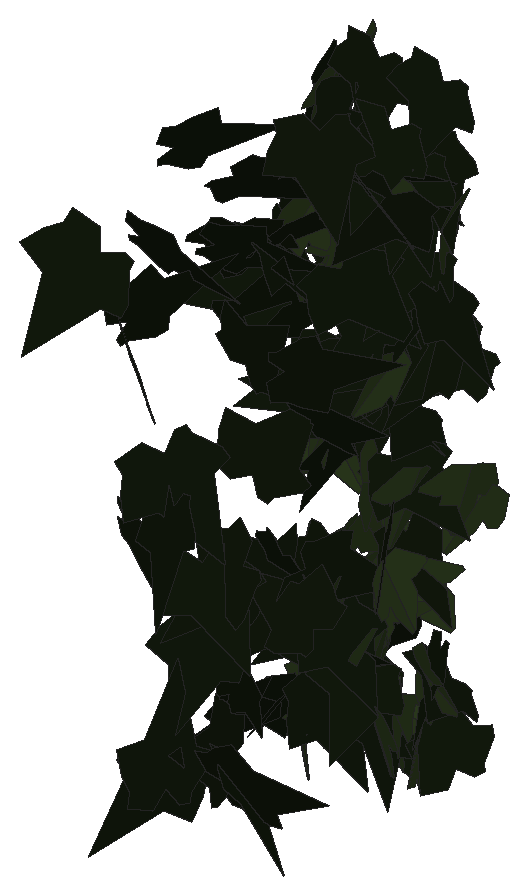
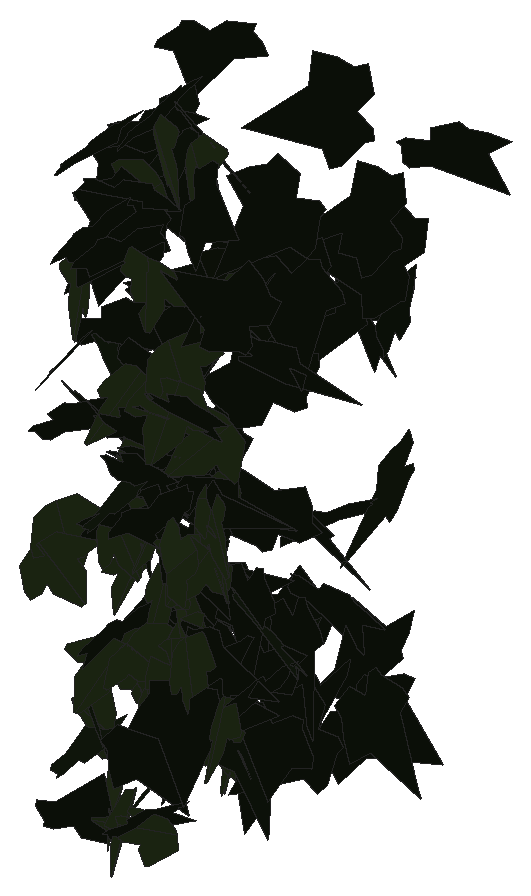
# SketchUp Ruby script. Lengths in inches.
U = 1.inch
M = Sketchup.active_model
def pt(a) = Geom::Point3d.new(a.map { |v| v * U })
def face(e, loops, mat)
  f = e.add_face(loops[0].map { |a| pt(a) })
  loops[1..].each { |l| e.add_face(l.map { |a| pt(a) }).erase! }
  f.material = f.back_material = mat if mat
  f
end
# faces: each face lists its corners as indices into pts; further lists are holes
def faces(e, pts, list, mat = nil) = list.each { |f| face(e, (f[0].is_a?(Array) ? f : [f]).map { |l| l.map { |i| pts[i] } }, mat) }
# xy, xz, yz: faces in a plane at the given z, y or x. An outline is a flat list of corners, or four numbers for a rectangle; further outlines are holes
def ring(l) = l.size == 4 ? [[l[0], l[1]], [l[2], l[1]], [l[2], l[3]], [l[0], l[3]]] : l.each_slice(2).to_a
def flat(e, list, mat, &to3) = list.each { |f| face(e, (f[0].is_a?(Array) ? f : [f]).map { |l| ring(l).map { |u, v| to3.(u, v) } }, mat) }
def xy(e, z, list, mat = nil) = flat(e, list, mat) { |x, y| [x, y, z] }
def xz(e, y, list, mat = nil) = flat(e, list, mat) { |x, z| [x, y, z] }
def yz(e, x, list, mat = nil) = flat(e, list, mat) { |y, z| [x, y, z] }
def lines(e, pts, list) = list.each { |a, b| e.add_line(pt(pts[a]), pt(pts[b])) }
# prism: a flat outline (further loops are holes) pulled along v
def prism(e, loops, v, mat = nil)
  f = face(e, loops, mat); d = Geom::Vector3d.new(v.map { |x| x * U })
  f.pushpull(f.normal.samedirection?(d) ? d.length : -d.length)
end
def box(e, o, s, mat = nil) = prism(e, [[o, [o[0] + s[0], o[1], o[2]], [o[0] + s[0], o[1] + s[1], o[2]], [o[0], o[1] + s[1], o[2]]]], [0, 0, s[2]], mat)
def at(x, y, z, deg = 0) = Geom::Transformation.translation(pt([x, y, z])) * Geom::Transformation.rotation(ORIGIN, Z_AXIS, deg.degrees)
def axes(o, x, y, z) = Geom::Transformation.new([*x, 0, *y, 0, *z, 0, *pt(o).to_a, 1])
def part(name) = M.definitions.add(name)
# library, detail: a bought-in or finely detailed component or shape, given as its bounding box
def library(name, o, s) = part(name).tap { |d| box(d.entities, o, s) }
def detail(e, o, s) = box(e.add_group.entities, o, s)
def put(e, d, t, mat = nil) = e.add_instance(d, t).tap { |i| i.material = mat if mat }
def group(e, t, mat = nil) = e.add_group.tap { |g| g.transformation = t; g.material = mat if mat }.entities
root = M.entities
M.materials.add("efeu1").color = [18, 25, 13]
M.materials.add("efeu2").color = [43, 57, 29]
c1 = part("ivyleaf_9")
p = [[1.54,2.16,1.25],[1.36,2.04,1.19],[-0.21,0.99,0.68],[-0.71,1.11,0.82],[-0.85,0.86,0.67],[-0.8,0.17,0.21],
  [-0.9,-0.01,0.1],[-0.67,-0.16,-0.02],[-0.08,-0.08,-0.05],[-0.03,-0.6,-0.4],[0.65,-0.88,-0.66],[0.83,-0.6,-0.49],
  [1.29,-0.42,-0.43],[1.8125,-0.07,-0.26],[1.21,0.44,0.15]]
faces(c1.entities,p,[[0,1,2,3,4,5,6,7,8,9,10,11,12,13,14]],"efeu1")
c2 = part("ivyleaf_10")
p = [[0,0.5,-0.03],[-0.0625,2.02,-0.43],[-0.19,2.01,-0.46],[-0.54,1.05,-0.29],[-0.52,0.625,-0.18],[-0.83,0.76,-0.28],
  [-1.16,0.64,-0.33],[-1.15,0.33,-0.24],[-0.77,-0.39,0.02],[-0.3,-0.51,0.16],[0.04,-0.48,0.23],[-0.02,2.01,-0.4375],
  [-0.06,2.01,-0.43],[0.04,-0.49,0.23],[0.67,-0.49,0.14],[1.38,0.36,-0.2],[1.375,0.51,-0.24],[0.81,0.65,-0.19],
  [0.62,0.59,-0.15],[0.6,1.09,-0.28],[0.5,1.23,-0.31]]
faces(c2.entities,p,[[0,1,2,3,4,5,6,7,8,9,10],[11,12,0,13,14,15,16,17,18,19,20]],"efeu2")
put(root,c1,axes([592.36,120.74,293.89],[-1.14457,0.06612,0.67883],[-0.67994,-0.00656,-1.1458],[-0.05352,-1.33072,0.03938]))
put(root,c1,axes([591.87,115.34,278.18],[-0.6134,1.00067,-0.76076],[0.3582,-0.67226,-1.17308],[-1.2049,-0.70929,0.03855]))
put(root,c2,axes([591.48,123.75,281.43],[0.25817,-0.97901,-0.59637],[0.14023,0.63368,-0.97957],[1.13774,0.14405,0.25606]))
put(root,c1,axes([591.9,111.61,298.5625],[-1.18923,-0.86005,0.10812],[-0.0968,-0.05064,-1.46755],[0.86139,-1.19306,-0.01565]))
put(root,c1,axes([592.14,119.23,296.43],[0.51316,1.03145,-0.63629],[-0.3835,-0.51727,-1.1478],[-1.14964,0.63295,0.09887]))
put(root,c1,axes([591.57,113.87,286.72],[1.18466,-0.50835,-0.63513],[-0.54554,0.33587,-1.28639],[0.60348,1.30154,0.0839]))
put(root,c1,axes([591.44,121.65,281.75],[0.54465,-0.90417,-0.67064],[-0.09148,0.707,-1.02748],[1.12201,0.49655,0.24178]))
put(root,c2,axes([592.77,122.97,288.59],[-0.65154,0.23488,0.97689],[-0.93643,0.27996,-0.69187],[-0.3641,-1.14036,0.03135]))
put(root,c1,axes([591.52,114.32,292.64],[-0.12498,-0.22861,1.35165],[0.38183,-1.30935,-0.18615],[1.3166,0.35803,0.18229]))
put(root,c1,axes([591.53,114.03,294.93],[0.43693,0.10982,1.41408],[1.05683,0.96162,-0.40122],[-0.94593,1.12509,0.2049]))
put(root,c1,axes([591.1,115.33,297.37],[1.16534,-0.32839,0.64756],[0.62053,-0.18536,-1.2107],[0.37699,1.32023,-0.00891]))
put(root,c1,axes([593.18,119.35,282.35],[-0.20471,0.90108,1.06087],[-0.70737,0.85614,-0.86368],[-1.19876,-0.65907,0.32848]))
put(root,c1,axes([592.625,114.95,277.32],[-0.06744,0.31516,-1.46174],[0.27376,-1.43589,-0.32222],[-1.47005,-0.28185,0.00705]))
put(root,c1,axes([593.2,123.18,289.14],[-1.02742,-0.18444,0.70049],[-0.69258,-0.10601,-1.04374],[0.21221,-1.23897,-0.01497]))
put(root,c2,axes([591.92,123.57,292.27],[-0.92808,-0.1007,-0.77885],[0.7694,0.12508,-0.93299],[0.15741,-1.20511,-0.03175]))
put(root,c1,axes([593.57,123.0625,288.75],[-0.81472,0.12778,0.98929],[-0.98397,0.10681,-0.82414],[-0.16381,-1.27713,0.03006]))
put(root,c1,axes([591.71,122.29,296.16],[0.21451,-0.10207,1.20924],[1.18259,-0.25797,-0.23156],[0.27231,1.20072,0.05304]))
put(root,c1,axes([592.15,120.32,292.25],[1.19976,0.61452,0.39653],[-0.38139,-0.12432,1.34661],[0.62403,-1.25746,0.06065]))
put(root,c1,axes([593.01,124.67,293.53],[-1.18188,-0.31478,-0.11874],[0.12949,-0.0253,-1.22173],[0.31051,-1.18756,0.0575]))
put(root,c1,axes([591.82,118.57,295.94],[1.10946,0.20211,0.77368],[0.74065,0.23905,-1.12455],[-0.30143,1.33129,0.08447]))
put(root,c1,axes([592.5,117.51,277.72],[0.60087,0.91157,0.89309],[0.51767,0.72816,-1.09151],[-1.16644,0.79274,-0.02436]))
put(root,c2,axes([592.72,125.05,287.43],[-0.29165,0.09054,-1.21967],[-0.07384,-1.25289,-0.07535],[-1.2208,0.05415,0.29594]))
put(root,c1,axes([593.89,122.01,282.14],[-0.5819,-0.01429,-1.14079],[-1.0494,-0.49574,0.5415],[-0.44762,1.18078,0.21353]))
put(root,c1,axes([593.09,123.7,281.29],[0.50094,1.04363,-0.38049],[-0.22491,-0.31346,-1.15588],[-1.08783,0.5454,0.06376]))
put(root,c1,axes([592.72,123.72,301.26],[-0.39489,0.23985,-1.23143],[0.90932,-0.83472,-0.45418],[-0.86435,-0.98773,0.08479]))
put(root,c2,axes([593.03,122.72,287.51],[0.92844,-0.7396,-0.28525],[-0.22808,0.17149,-1.18699],[0.75918,0.95601,-0.00776]))
put(root,c2,axes([592.6875,123.07,289.2],[-0.19418,-0.48725,1.13069],[0.48465,-1.0825,-0.38325],[1.13181,0.37994,0.3581]))
put(root,c1,axes([593,119.29,278.41],[0.68816,1.04968,-0.22079],[-0.12979,-0.17891,-1.25511],[-1.06477,0.70022,0.01029]))
put(root,c2,axes([593.11,121.79,296.25],[0.17074,0.86733,-0.87553],[-0.36793,-0.8077,-0.87189],[-1.17619,0.37857,0.14565]))
put(root,c1,axes([592.42,119.75,286.65],[-0.59776,0.14735,1.18784],[1.15522,-0.27647,0.61564],[0.31327,1.30071,-0.00371]))
put(root,c1,axes([592.6875,118.47,299.01],[0.91336,0.85435,0.43133],[0.28933,0.32184,-1.25016],[-0.91227,0.95744,0.03535]))
put(root,c1,axes([592.35,115.6,301.36],[0.77511,0.32705,1.07998],[0.86109,0.67535,-0.82253],[-0.72929,1.14501,0.17667]))
put(root,c1,axes([593.62,119.91,278.14],[-0.40094,1.2023,0.0323],[-0.01282,0.02977,-1.26739],[-1.20266,-0.40114,0.00274]))
put(root,c1,axes([592.77,120.47,295.85],[0.78154,-0.78906,-0.71759],[-0.42743,0.58335,-1.10696],[0.97717,0.88625,0.08972]))
put(root,c1,axes([593.46,122.84,280.26],[-0.04447,-0.31006,-1.22847],[0.30591,-1.19549,0.29066],[-1.22951,-0.28623,0.11675]))
put(root,c2,axes([593.42,123.23,282.82],[0.01057,-1.23367,-0.11013],[0.01481,0.11025,-1.23362],[1.23849,0.00921,0.01569]))
put(root,c1,axes([593.21,119.91,296.04],[0.67149,0.8277,0.75502],[0.24329,0.75151,-1.04022],[-1.09359,0.67541,0.23218]))
put(root,c1,axes([593.42,115.95,282.15],[-1.19994,-0.5015,-0.53202],[0.54584,0.06578,-1.29311],[0.48642,-1.31095,0.13864]))
put(root,c2,axes([592.8,123.29,286.86],[0.89368,0.46056,0.67156],[0.54269,0.40653,-1.00099],[-0.60711,1.04134,0.09377]))
put(root,c1,axes([592.92,119.89,281.55],[-0.04048,-0.64148,-1.07577],[0.18545,1.0614,-0.63989],[1.2387,-0.17987,0.06064]))
put(root,c2,axes([593.4,124.21,293.43],[-1.05983,-0.54132,-0.28818],[0.26753,0.10963,-1.18984],[0.55181,-1.09282,0.02338]))
put(root,c1,axes([593.83,119.51,283.83],[0.75895,0.12806,-1.02845],[-1.01927,-0.1385,-0.76942],[-0.18759,1.27064,0.01978]))
put(root,c2,axes([593.74,123.67,294.68],[-0.45042,-1.10615,0.30759],[-0.0669,-0.30457,-1.19324],[1.14617,-0.45247,0.05123]))
put(root,c1,axes([593.65,116.82,277.02],[-0.16039,-0.16384,1.30254],[-0.52908,-1.19287,-0.21519],[1.20147,-0.54717,0.07912]))
put(root,c1,axes([594.23,116.5,280.97],[0.60896,0.08753,-1.29393],[-1.28109,-0.18182,-0.61522],[-0.20179,1.41846,0.00099]))
put(root,c1,axes([593.78,113.13,277.63],[-0.54837,-0.83607,1.09748],[0.7088,0.84251,0.99599],[-1.18368,0.89183,0.08796]))
put(root,c1,axes([593.99,122.47,287.18],[-0.27911,0.9267,-0.67379],[0.18658,-0.64747,-0.96779],[-1.13046,-0.33566,0.00662]))
put(root,c2,axes([593.8125,122.24,301.8],[0.28246,-1.20475,0.05693],[-0.00345,-0.05928,-1.23731],[1.20609,0.28197,-0.01687]))
put(root,c1,axes([594.1875,123.58,289.55],[-0.71191,-0.79199,0.51244],[-0.37642,-0.35015,-1.06412],[0.86495,-0.80424,-0.04133]))
put(root,c1,axes([594.66,116.08,285.22],[-1.41106,0.21487,-0.05452],[0.05394,-0.00797,-1.42733],[-0.21502,-1.41209,-0.00024]))
put(root,c2,axes([594.67,120.52,278.25],[0.78121,-0.22671,-0.94822],[-0.88273,0.35136,-0.81126],[0.41389,1.17727,0.05952]))
put(root,c2,axes([594.11,120.05,277.58],[-0.69502,0.87875,-0.32007],[0.13699,-0.29883,-1.11787],[-0.92514,-0.70441,0.07493]))
put(root,c1,axes([593.54,115.5625,285.07],[0.10712,-1.33487,-0.47382],[0.48344,0.4811,-1.24607],[1.33141,-0.06729,0.49058]))
put(root,c1,axes([594.1,124.49,288.97],[-0.38033,-1.20414,-0.13162],[0.02716,0.12944,-1.26271],[1.21101,-0.38108,-0.01302]))
put(root,c1,axes([593.6875,117.73,292.3],[-0.32433,0.02926,1.27197],[0.87949,-0.94337,0.24596],[0.91938,0.91277,0.21343]))
put(root,c2,axes([594.63,122.64,282.09],[-0.24481,-1.18275,-0.22608],[0.01441,0.22781,-1.20741],[1.20408,-0.2432,-0.03152]))
put(root,c2,axes([594.54,123.34,302.76],[0.61918,-1.08302,0.07791],[0.02767,-0.07392,-1.24746],[1.08547,0.61967,-0.01264]))
put(root,c1,axes([595.07,124.08,279.53],[-0.3421,0.84605,-0.72768],[0.08107,-0.74025,-0.89878],[-1.11299,-0.31397,0.1582]))
put(root,c1,axes([594.78,124.73,276.42],[-0.74029,-0.78602,0.47071],[-0.1117,-0.52322,-1.04938],[0.90935,-0.70416,0.2543]))
put(root,c1,axes([595.23,124.16,290.58],[-1.12016,-0.20027,0.3169],[-0.24984,-0.34563,-1.10155],[0.27949,-1.11163,0.2854]))
put(root,c1,axes([595.16,124.66,292.2],[-1.05773,-0.53843,0.06073],[-0.04621,-0.04308,-1.18676],[0.53987,-1.0586,0.01741]))
put(root,c2,axes([595.33,122.21,281.22],[-0.98025,0.27387,0.58187],[-0.55504,0.17549,-1.01765],[-0.32483,-1.12635,-0.01707]))
put(root,c2,axes([594.98,124.3,283.04],[0.44656,0.84491,-0.76393],[-0.35323,-0.67737,-0.95566],[-1.08291,0.56937,-0.0033]))
put(root,c1,axes([595.34,124.28,290.17],[-1.15934,-0.2236,-0.0257],[0.02457,0.00828,-1.1807],[0.22373,-1.15959,-0.00348]))
put(root,c1,axes([595.125,121.53,282.52],[-1.10779,-0.30583,-0.39696],[0.3785,0.12054,-1.14914],[0.3284,-1.17058,-0.01463]))
put(root,c2,axes([594.21,123.96,275.89],[0.11159,-0.35015,-1.1133],[1.16266,0.13053,0.07548],[0.10141,-1.11124,0.35967]))
put(root,c2,axes([595.27,121.73,281.9],[0.18955,0.7399,-0.97327],[-0.30465,-0.92525,-0.76273],[-1.18402,0.35651,0.04044]))
put(root,c1,axes([596.17,118.125,282.54],[-0.26181,0.40964,1.0866],[-1.07681,0.33134,-0.38436],[-0.43472,-1.06746,0.29768]))
put(root,c2,axes([595.28,122.19,284.69],[0.00129,-0.96061,-0.67602],[0.1165,0.67279,-0.9558],[1.16884,-0.066,0.09601]))
put(root,c1,axes([594.85,120.42,278.64],[0.37256,-1.10985,-0.79003],[-0.27047,0.74248,-1.17059],[1.3352,0.46008,-0.01669]))
put(root,c1,axes([596.2,122.03,292.17],[-0.0149,0.32803,1.17932],[-1.15596,0.38422,-0.12148],[-0.40269,-1.11507,0.30508]))
put(root,c1,axes([594.31,120.11,280.37],[0.7151,0.43704,-0.94075],[0.82744,0.44877,0.83746],[0.62559,-1.09316,-0.03231]))
put(root,c1,axes([594.33,120.6,288.99],[0.38034,-0.47525,1.13365],[1.05355,-0.48532,-0.55693],[0.63328,1.09283,0.24567]))
put(root,c2,axes([595.47,120.74,282.82],[0.40277,-1.1928,0.12568],[0.03865,-0.1196,-1.25897],[1.19878,0.40461,-0.00163]))
put(root,c1,axes([596.05,120.27,302.02],[-1.243,0.36607,-0.1268],[0.11786,-0.04862,-1.29571],[-0.36904,-1.2485,0.01328]))
put(root,c1,axes([595,111.65,291.64],[0.04716,-1.06233,-1.02471],[0.12233,1.02452,-1.0565],[1.47092,-0.05114,0.12072]))
put(root,c2,axes([595.33,123.01,297.26],[1.23408,0.00638,0.19622],[0.1933,0.17878,-1.22154],[-0.0343,1.23673,0.17557]))
put(root,c2,axes([595.8125,122.18,279.71],[0.14084,-1.20988,0.01144],[0.00659,-0.01075,-1.21804],[1.20992,0.1409,0.00531]))
put(root,c1,axes([595.32,119.18,284.02],[0.18789,0.1676,-1.27506],[-0.09623,1.28682,0.15497],[1.28242,0.072,0.19844]))
put(root,c2,axes([595.92,123.53,276.19],[-0.39301,1.02545,0.52096],[-0.30772,0.43672,-1.09178],[-1.10826,-0.4849,0.11841]))
put(root,c2,axes([595.92,123.13,290.6875],[0.11813,0.57585,-1.08771],[-0.26817,-1.05441,-0.58734],[-1.20117,0.29204,0.02415]))
put(root,c2,axes([595.96,121.51,286.76],[0.30336,-0.50496,-1.11947],[0.02076,1.15506,-0.51539],[1.22791,0.10523,0.28528]))
put(root,c2,axes([595.67,123.6,292.86],[-0.23598,-0.78626,-0.90793],[0.4662,0.79277,-0.80771],[1.10688,-0.50153,0.14663]))
put(root,c1,axes([595.57,122.61,276.62],[0.23939,-1.14543,0.32709],[0.13089,-0.30632,-1.16848],[1.184,0.26546,0.06304]))
put(root,c1,axes([595.58,120.78,295.2],[-0.07969,-0.47823,-1.25039],[0.29622,1.21525,-0.48368],[1.30554,-0.30493,0.03342]))
put(root,c1,axes([595.77,122.36,302.97],[-0.05535,-1.23831,0.35809],[0.04466,-0.36005,-1.23817],[1.28827,-0.04072,0.05831]))
put(root,c1,axes([595.93,110.78,290.2],[-0.96955,-0.06355,-1.07431],[1.07602,-0.03196,-0.96921],[0.01882,-1.44677,0.0686]))
put(root,c1,axes([595.84,124.49,288.32],[-0.32102,-0.91042,0.83619],[0.25913,-0.89429,-0.8742],[1.20869,-0.05008,0.4095]))
put(root,c1,axes([595.92,123.87,283.5],[0.3791,-1.02551,-0.53719],[-0.06728,0.54478,-1.08749],[1.15573,0.3681,0.1129]))
put(root,c2,axes([595.96,122.14,281.74],[0.01845,-0.3794,-1.17494],[0.79132,0.90563,-0.28001],[0.94775,-0.74877,0.25667]))
put(root,c1,axes([595.68,114.67,278.05],[0.82191,-1.09433,0.36045],[0.19321,-0.30559,-1.36832],[1.13585,0.84384,-0.02807]))
put(root,c1,axes([596.18,119.62,282.07],[0.04979,-0.9833,-0.74105],[0.03747,0.74252,-0.98273],[1.2307,0.01718,0.0599]))
put(root,c1,axes([596.29,123.41,298.18],[-0.12087,-1.09468,-0.56798],[0.06914,0.56379,-1.10132],[1.23132,-0.13911,0.00609]))
put(root,c1,axes([597.31,122.63,293.34],[-0.93964,0.84628,-0.01275],[0.00968,-0.00831,-1.26456],[-0.84632,-0.93969,-0.0003]))
put(root,c1,axes([596.87,123.58,295.11],[-0.83928,-0.89633,0.20818],[-0.16022,-0.13512,-1.22769],[0.90613,-0.8541,-0.02425]))
put(root,c2,axes([596.41,123.63,281.95],[0.63924,0.72765,0.69517],[0.23449,0.69319,-0.9412],[-0.97864,0.64139,0.22856]))
put(root,c2,axes([596.81,120.93,280.79],[0.2623,-1.00435,0.55414],[0.25075,-0.50449,-1.03306],[1.11934,0.34837,0.10157]))
put(root,c2,axes([597.07,122.66,286.56],[-0.08654,-1.15633,0.42915],[0.07674,-0.43442,-1.15505],[1.231,-0.0542,0.10218]))
put(root,c1,axes([597.09,120.25,280.12],[-0.66371,-1.0191,0.02927],[-0.02011,-0.02184,-1.21617],[1.01933,-0.66399,-0.00493]))
put(root,c2,axes([596.75,123.44,275.57],[-0.09811,0.15125,-1.11877],[0.31922,-1.07344,-0.17311],[-1.08288,-0.33014,0.05033]))
put(root,c1,axes([596.76,121.88,298.64],[1.08737,0.67683,0.16824],[0.12203,0.12217,-1.28022],[-0.68667,1.0935,0.0389]))
put(root,c1,axes([596.49,122.71,287.1875],[0.36574,-0.87243,-0.82538],[0.21077,0.89604,-0.85372],[1.18236,0.11014,0.40751]))
put(root,c1,axes([596.3,116.83,293.25],[0.51007,0.70814,-1.0652],[0.45088,0.97362,0.86317],[1.197,-0.6685,0.12878]))
put(root,c1,axes([596.83,124.23,299.01],[0.145,-1.21425,-0.24147],[-0.02921,0.2397,-1.22288],[1.23768,0.14791,-0.00057]))
put(root,c1,axes([597.81,124.03,275.02],[-1.1371,-0.42775,0.18167],[0.1954,-0.00435,1.21275],[-0.42166,1.15151,0.07207]))
put(root,c1,axes([597.75,123.68,291.62],[-1.21628,0.04784,-0.31719],[0.30781,-0.17592,-1.20687],[-0.09027,-1.24459,0.1584]))
put(root,c1,axes([596.74,119.32,300.76],[1.25666,-0.52278,-0.12136],[-0.11193,0.0469,-1.36107],[0.52488,1.26164,0.00031]))
put(root,c1,axes([596.24,113.78,278.13],[0.55442,-0.43722,1.30787],[1.22311,-0.49516,-0.68402],[0.63694,1.33143,0.1751]))
put(root,c2,axes([597.9375,123.53,296.42],[-0.04854,0.68487,0.99138],[-0.7436,0.76369,-0.56398],[-0.94812,-0.63401,0.39157]))
put(root,c1,axes([597.48,120.82,301.38],[-0.71967,-1.05973,-0.05846],[0.03878,0.04433,-1.28098],[1.06064,-0.72068,0.00717]))
put(root,c2,axes([597.51,120.1,278.58],[-0.96106,0.69561,-0.02515],[0.02077,-0.0142,-1.18639],[-0.69575,-0.96129,-0.00068]))
put(root,c1,axes([597.43,123.64,279.45],[-0.78436,0.16839,-0.8535],[0.82143,-0.23508,-0.80127],[-0.28648,-1.13509,0.03933]))
put(root,c1,axes([597.43,122.26,299.41],[-0.88601,-0.83086,-0.43582],[0.38089,0.22929,-1.21146],[0.85743,-0.96041,0.08781]))
put(root,c1,axes([597.32,123.95,301.87],[-0.28803,-1.14377,0.45283],[0.06067,-0.47772,-1.16804],[1.22865,-0.24454,0.16383]))
put(root,c2,axes([597.04,121.01,298.99],[-0.87502,0.28806,-0.84956],[0.81263,-0.24813,-0.92111],[-0.37995,-1.19408,-0.01354]))
put(root,c1,axes([597.27,124.45,278.05],[-0.34564,-0.82107,0.78571],[0.33731,-0.85835,-0.7486],[1.08523,0.00529,0.48292]))
put(root,c1,axes([598,124.8,291.26],[-0.81732,-0.66662,0.5649],[-0.32431,-0.48682,-1.04371],[0.81136,-0.8661,0.15187]))
put(root,c1,axes([598.32,119.85,299.54],[0.39525,0.52275,-1.20226],[-0.66363,-1.00316,-0.65436],[-1.13061,0.77157,-0.03622]))
put(root,c1,axes([597.43,120.88,285.72],[-0.25252,-0.17771,-1.14255],[1.09221,-0.42056,-0.17598],[-0.37957,-1.09193,0.25373]))
put(root,c1,axes([597.66,116.82,303.13],[-0.47432,-0.99512,-0.72011],[0.3171,0.64657,-1.10236],[1.18671,-0.57051,0.00674]))
put(root,c2,axes([597.14,123.125,278.67],[-0.02098,-0.11471,1.23716],[1.21745,-0.24892,-0.00244],[0.24805,1.21204,0.11659]))
put(root,c2,axes([597.91,120.41,284.12],[-0.06261,1.13127,0.37431],[-0.00622,0.37451,-1.13292],[-1.19157,-0.0614,-0.01375]))
put(root,c2,axes([598.46,124.71,285.62],[-0.59475,-0.77398,0.67122],[-0.17978,-0.68524,-0.94944],[1.00859,-0.57854,0.22658]))
put(root,c2,axes([598.55,123.9,286.76],[-0.51338,-1.07875,0.23056],[-0.06877,-0.22251,-1.19423],[1.10097,-0.51692,0.03291]))
put(root,c1,axes([597.89,123.18,293.99],[0.65756,-1.008,-0.38591],[-0.05573,0.41957,-1.1909],[1.07791,0.63661,0.17384]))
